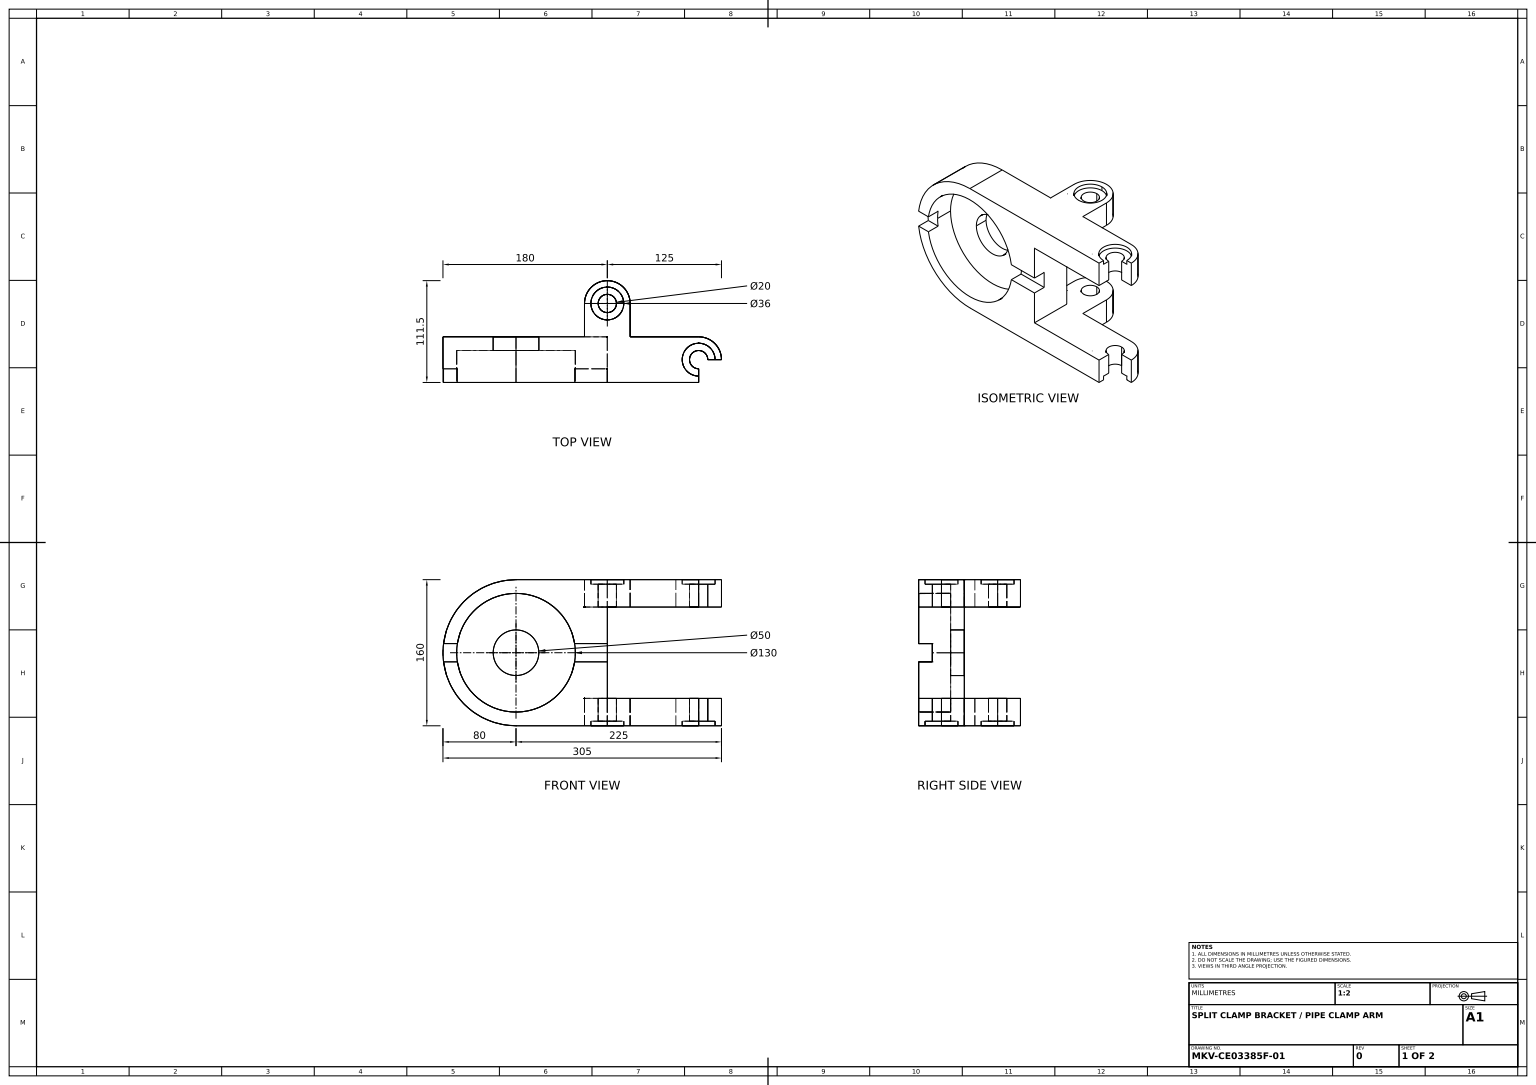
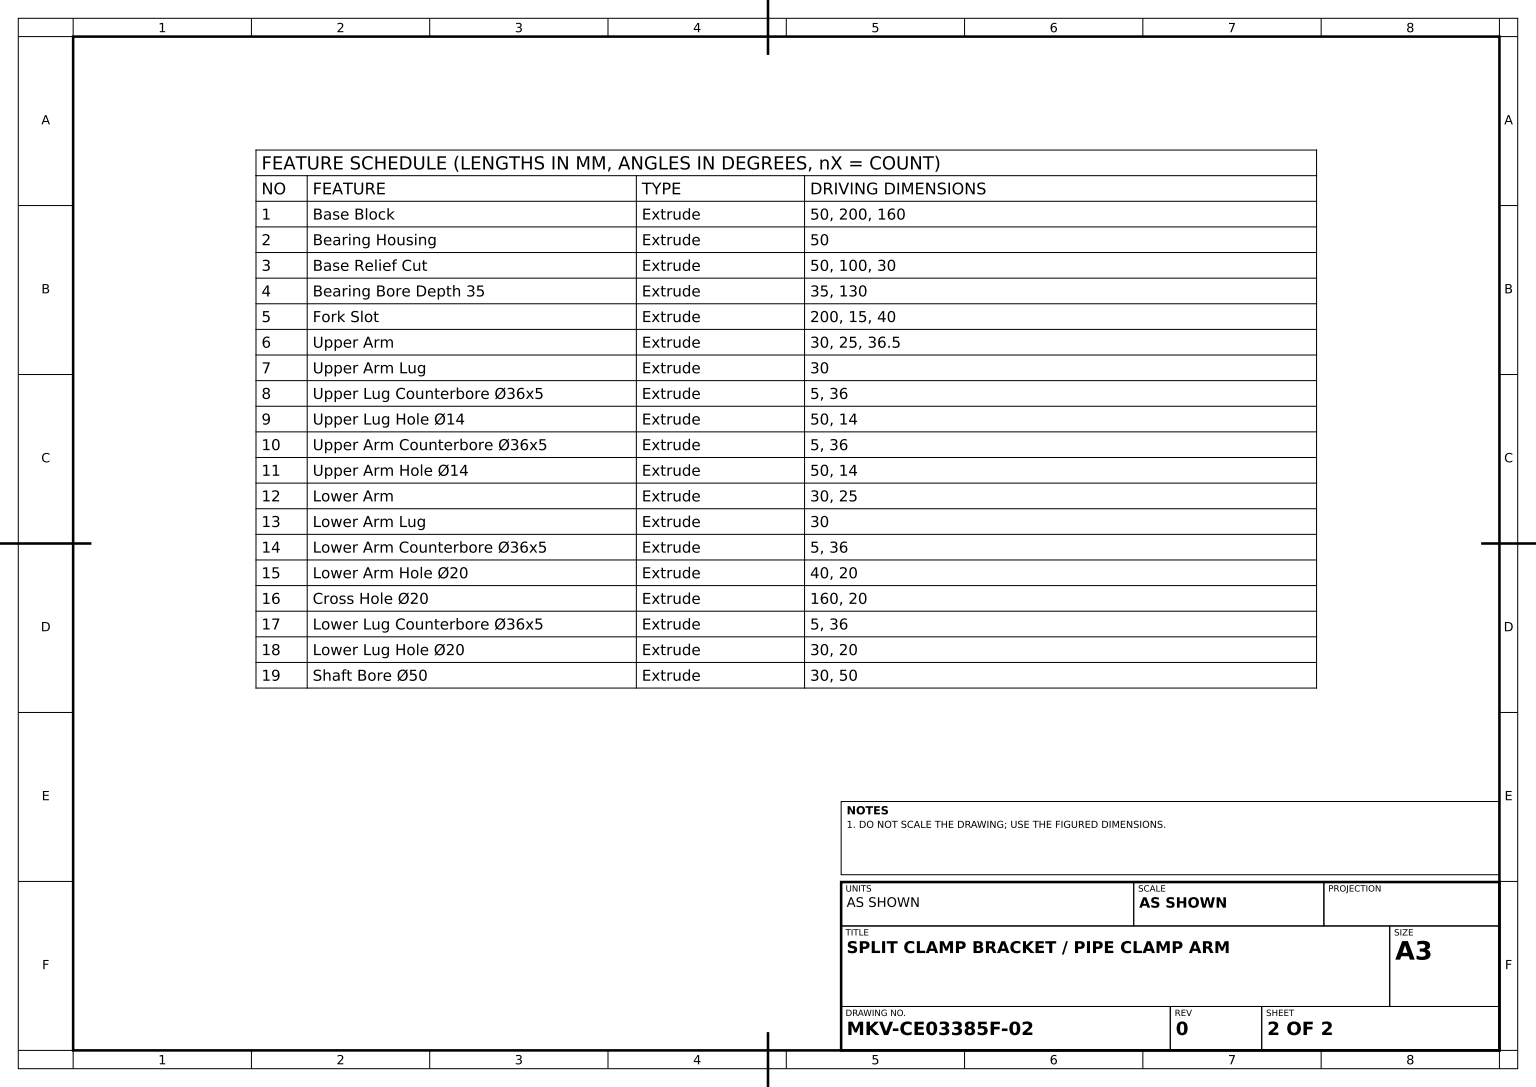
ISO-10303-21;
HEADER;
FILE_DESCRIPTION((''),'2;1');
FILE_NAME('','',(''),(''),'','','');
FILE_SCHEMA(('AUTOMOTIVE_DESIGN'));
ENDSEC;
DATA;
#1=APPLICATION_CONTEXT('');
#2=PRODUCT_CONTEXT('',#1,'mechanical');
#3=PRODUCT('','','',(#2));
#4=PRODUCT_DEFINITION_FORMATION('','',#3);
#5=PRODUCT_DEFINITION_CONTEXT('',#1,'design');
#6=PRODUCT_DEFINITION('','',#4,#5);
#7=PRODUCT_DEFINITION_SHAPE('','',#6);
#8=(LENGTH_UNIT()NAMED_UNIT(*)SI_UNIT(.MILLI.,.METRE.));
#9=(NAMED_UNIT(*)PLANE_ANGLE_UNIT()SI_UNIT($,.RADIAN.));
#10=(NAMED_UNIT(*)SI_UNIT($,.STERADIAN.)SOLID_ANGLE_UNIT());
#11=UNCERTAINTY_MEASURE_WITH_UNIT(LENGTH_MEASURE(1.E-05),#8,'distance_accuracy_value','');
#12=(GEOMETRIC_REPRESENTATION_CONTEXT(3)GLOBAL_UNCERTAINTY_ASSIGNED_CONTEXT((#11))GLOBAL_UNIT_ASSIGNED_CONTEXT((#8,#9,#10))REPRESENTATION_CONTEXT('',''));
#13=CARTESIAN_POINT('',(100.,130.,-26.5));
#14=VERTEX_POINT('',#13);
#15=CARTESIAN_POINT('',(100.,130.,-46.5));
#16=VERTEX_POINT('',#15);
#17=CARTESIAN_POINT('',(100.,130.,-36.5));
#18=DIRECTION('',(0.,1.,0.));
#19=DIRECTION('',(0.,0.,1.));
#20=AXIS2_PLACEMENT_3D('',#17,#18,#19);
#21=CIRCLE('',#20,10.);
#22=EDGE_CURVE('',#14,#16,#21,.T.);
#23=ORIENTED_EDGE('',*,*,#22,.T.);
#24=EDGE_CURVE('',#16,#14,#21,.T.);
#25=ORIENTED_EDGE('',*,*,#24,.T.);
#26=EDGE_LOOP('',(#23,#25));
#27=FACE_BOUND('',#26,.T.);
#28=CARTESIAN_POINT('',(100.,130.,0.));
#29=VERTEX_POINT('',#28);
#30=CARTESIAN_POINT('',(100.,130.,50.));
#31=VERTEX_POINT('',#30);
#32=VECTOR('',#19,1000.);
#33=LINE('',#28,#32);
#34=EDGE_CURVE('',#29,#31,#33,.T.);
#35=ORIENTED_EDGE('',*,*,#34,.F.);
#36=CARTESIAN_POINT('',(75.,130.,0.));
#37=VERTEX_POINT('',#36);
#38=CARTESIAN_POINT('',(125.,130.,0.));
#39=DIRECTION('',(1.,0.,0.));
#40=VECTOR('',#39,1000.);
#41=LINE('',#38,#40);
#42=EDGE_CURVE('',#37,#29,#41,.T.);
#43=ORIENTED_EDGE('',*,*,#42,.F.);
#44=CARTESIAN_POINT('',(75.,130.,-36.5));
#45=VERTEX_POINT('',#44);
#46=LINE('',#44,#32);
#47=EDGE_CURVE('',#45,#37,#46,.T.);
#48=ORIENTED_EDGE('',*,*,#47,.F.);
#49=CARTESIAN_POINT('',(125.,130.,-36.5));
#50=VERTEX_POINT('',#49);
#51=CIRCLE('',#20,25.);
#52=EDGE_CURVE('',#50,#45,#51,.T.);
#53=ORIENTED_EDGE('',*,*,#52,.F.);
#54=VERTEX_POINT('',#38);
#55=DIRECTION('',(0.,0.,-1.));
#56=VECTOR('',#55,1000.);
#57=LINE('',#49,#56);
#58=EDGE_CURVE('',#54,#50,#57,.T.);
#59=ORIENTED_EDGE('',*,*,#58,.F.);
#60=CARTESIAN_POINT('',(200.,130.,0.));
#61=VERTEX_POINT('',#60);
#62=DIRECTION('',(-1.,0.,0.));
#63=VECTOR('',#62,1000.);
#64=LINE('',#60,#63);
#65=EDGE_CURVE('',#61,#54,#64,.T.);
#66=ORIENTED_EDGE('',*,*,#65,.F.);
#67=CARTESIAN_POINT('',(225.,130.,25.));
#68=VERTEX_POINT('',#67);
#69=CARTESIAN_POINT('',(200.,130.,25.));
#70=AXIS2_PLACEMENT_3D('',#69,#18,#19);
#71=CIRCLE('',#70,25.);
#72=EDGE_CURVE('',#68,#61,#71,.T.);
#73=ORIENTED_EDGE('',*,*,#72,.F.);
#74=CARTESIAN_POINT('',(210.,130.,25.));
#75=VERTEX_POINT('',#74);
#76=LINE('',#69,#40);
#77=EDGE_CURVE('',#75,#68,#76,.T.);
#78=ORIENTED_EDGE('',*,*,#77,.F.);
#79=CARTESIAN_POINT('',(200.,130.,35.));
#80=VERTEX_POINT('',#79);
#81=CIRCLE('',#70,10.);
#82=EDGE_CURVE('',#75,#80,#81,.T.);
#83=ORIENTED_EDGE('',*,*,#82,.T.);
#84=CARTESIAN_POINT('',(200.,130.,50.));
#85=VERTEX_POINT('',#84);
#86=LINE('',#60,#32);
#87=EDGE_CURVE('',#80,#85,#86,.T.);
#88=ORIENTED_EDGE('',*,*,#87,.T.);
#89=LINE('',#84,#63);
#90=EDGE_CURVE('',#85,#31,#89,.T.);
#91=ORIENTED_EDGE('',*,*,#90,.T.);
#92=EDGE_LOOP('',(#35,#43,#48,#53,#59,#66,#73,#78,#83,#88,#91));
#93=FACE_OUTER_BOUND('',#92,.T.);
#94=AXIS2_PLACEMENT_3D('',#60,#18,#19);
#95=PLANE('',#94);
#96=ADVANCED_FACE('',(#27,#93),#95,.F.);
#97=ORIENTED_EDGE('',*,*,#52,.T.);
#98=CARTESIAN_POINT('',(75.,160.,-36.5));
#99=VERTEX_POINT('',#98);
#100=VECTOR('',#18,1000.);
#101=LINE('',#44,#100);
#102=EDGE_CURVE('',#45,#99,#101,.T.);
#103=ORIENTED_EDGE('',*,*,#102,.T.);
#104=CARTESIAN_POINT('',(125.,160.,-36.5));
#105=VERTEX_POINT('',#104);
#106=CARTESIAN_POINT('',(100.,160.,-36.5));
#107=AXIS2_PLACEMENT_3D('',#106,#18,#19);
#108=CIRCLE('',#107,25.);
#109=EDGE_CURVE('',#105,#99,#108,.T.);
#110=ORIENTED_EDGE('',*,*,#109,.F.);
#111=LINE('',#49,#100);
#112=EDGE_CURVE('',#50,#105,#111,.T.);
#113=ORIENTED_EDGE('',*,*,#112,.F.);
#114=EDGE_LOOP('',(#97,#103,#110,#113));
#115=FACE_OUTER_BOUND('',#114,.T.);
#116=CYLINDRICAL_SURFACE('',#20,25.);
#117=ADVANCED_FACE('',(#115),#116,.T.);
#118=CARTESIAN_POINT('',(200.,30.,0.));
#119=VERTEX_POINT('',#118);
#120=CARTESIAN_POINT('',(225.,30.,25.));
#121=VERTEX_POINT('',#120);
#122=CARTESIAN_POINT('',(200.,30.,25.));
#123=DIRECTION('',(0.,-1.,0.));
#124=AXIS2_PLACEMENT_3D('',#122,#123,#55);
#125=CIRCLE('',#124,25.);
#126=EDGE_CURVE('',#119,#121,#125,.T.);
#127=ORIENTED_EDGE('',*,*,#126,.T.);
#128=CARTESIAN_POINT('',(225.,0.,25.));
#129=VERTEX_POINT('',#128);
#130=VECTOR('',#123,1000.);
#131=LINE('',#120,#130);
#132=EDGE_CURVE('',#121,#129,#131,.T.);
#133=ORIENTED_EDGE('',*,*,#132,.T.);
#134=CARTESIAN_POINT('',(200.,0.,0.));
#135=VERTEX_POINT('',#134);
#136=CARTESIAN_POINT('',(200.,0.,25.));
#137=AXIS2_PLACEMENT_3D('',#136,#123,#55);
#138=CIRCLE('',#137,25.);
#139=EDGE_CURVE('',#135,#129,#138,.T.);
#140=ORIENTED_EDGE('',*,*,#139,.F.);
#141=LINE('',#134,#100);
#142=EDGE_CURVE('',#135,#119,#141,.T.);
#143=ORIENTED_EDGE('',*,*,#142,.T.);
#144=EDGE_LOOP('',(#127,#133,#140,#143));
#145=FACE_OUTER_BOUND('',#144,.T.);
#146=CYLINDRICAL_SURFACE('',#124,25.);
#147=ADVANCED_FACE('',(#145),#146,.T.);
#148=CARTESIAN_POINT('',(200.,5.,35.));
#149=VERTEX_POINT('',#148);
#150=CARTESIAN_POINT('',(200.,30.,35.));
#151=VERTEX_POINT('',#150);
#152=CARTESIAN_POINT('',(200.,45.,35.));
#153=LINE('',#152,#100);
#154=EDGE_CURVE('',#149,#151,#153,.T.);
#155=ORIENTED_EDGE('',*,*,#154,.T.);
#156=CARTESIAN_POINT('',(200.,30.,50.));
#157=VERTEX_POINT('',#156);
#158=LINE('',#118,#32);
#159=EDGE_CURVE('',#151,#157,#158,.T.);
#160=ORIENTED_EDGE('',*,*,#159,.T.);
#161=CARTESIAN_POINT('',(200.,0.,50.));
#162=VERTEX_POINT('',#161);
#163=LINE('',#161,#100);
#164=EDGE_CURVE('',#162,#157,#163,.T.);
#165=ORIENTED_EDGE('',*,*,#164,.F.);
#166=CARTESIAN_POINT('',(200.,0.,43.));
#167=VERTEX_POINT('',#166);
#168=LINE('',#161,#56);
#169=EDGE_CURVE('',#162,#167,#168,.T.);
#170=ORIENTED_EDGE('',*,*,#169,.T.);
#171=CARTESIAN_POINT('',(200.,5.,43.));
#172=VERTEX_POINT('',#171);
#173=LINE('',#171,#100);
#174=EDGE_CURVE('',#167,#172,#173,.T.);
#175=ORIENTED_EDGE('',*,*,#174,.T.);
#176=CARTESIAN_POINT('',(200.,5.,50.));
#177=LINE('',#176,#32);
#178=EDGE_CURVE('',#149,#172,#177,.T.);
#179=ORIENTED_EDGE('',*,*,#178,.F.);
#180=EDGE_LOOP('',(#155,#160,#165,#170,#175,#179));
#181=FACE_OUTER_BOUND('',#180,.T.);
#182=AXIS2_PLACEMENT_3D('',#161,#62,#19);
#183=PLANE('',#182);
#184=ADVANCED_FACE('',(#181),#183,.F.);
#185=CARTESIAN_POINT('',(-79.372539,70.,50.));
#186=VERTEX_POINT('',#185);
#187=CARTESIAN_POINT('',(0.,0.,50.));
#188=VERTEX_POINT('',#187);
#189=CARTESIAN_POINT('',(0.,80.,50.));
#190=AXIS2_PLACEMENT_3D('',#189,#19,#39);
#191=CIRCLE('',#190,80.);
#192=EDGE_CURVE('',#186,#188,#191,.T.);
#193=ORIENTED_EDGE('',*,*,#192,.F.);
#194=CARTESIAN_POINT('',(-79.372539,70.,35.));
#195=VERTEX_POINT('',#194);
#196=CARTESIAN_POINT('',(-79.372539,70.,0.));
#197=LINE('',#196,#32);
#198=EDGE_CURVE('',#195,#186,#197,.T.);
#199=ORIENTED_EDGE('',*,*,#198,.F.);
#200=CARTESIAN_POINT('',(-79.372539,90.,35.));
#201=VERTEX_POINT('',#200);
#202=CARTESIAN_POINT('',(0.,80.,35.));
#203=AXIS2_PLACEMENT_3D('',#202,#19,#62);
#204=CIRCLE('',#203,80.);
#205=EDGE_CURVE('',#201,#195,#204,.T.);
#206=ORIENTED_EDGE('',*,*,#205,.F.);
#207=CARTESIAN_POINT('',(-79.372539,90.,50.));
#208=VERTEX_POINT('',#207);
#209=CARTESIAN_POINT('',(-79.372539,90.,0.));
#210=LINE('',#209,#56);
#211=EDGE_CURVE('',#208,#201,#210,.T.);
#212=ORIENTED_EDGE('',*,*,#211,.F.);
#213=CARTESIAN_POINT('',(0.,160.,50.));
#214=VERTEX_POINT('',#213);
#215=EDGE_CURVE('',#214,#208,#191,.T.);
#216=ORIENTED_EDGE('',*,*,#215,.F.);
#217=CARTESIAN_POINT('',(0.,160.,0.));
#218=VERTEX_POINT('',#217);
#219=LINE('',#213,#56);
#220=EDGE_CURVE('',#214,#218,#219,.T.);
#221=ORIENTED_EDGE('',*,*,#220,.T.);
#222=CARTESIAN_POINT('',(0.,0.,0.));
#223=VERTEX_POINT('',#222);
#224=CARTESIAN_POINT('',(0.,80.,0.));
#225=AXIS2_PLACEMENT_3D('',#224,#19,#39);
#226=CIRCLE('',#225,80.);
#227=EDGE_CURVE('',#218,#223,#226,.T.);
#228=ORIENTED_EDGE('',*,*,#227,.T.);
#229=LINE('',#187,#56);
#230=EDGE_CURVE('',#188,#223,#229,.T.);
#231=ORIENTED_EDGE('',*,*,#230,.F.);
#232=EDGE_LOOP('',(#193,#199,#206,#212,#216,#221,#228,#231));
#233=FACE_OUTER_BOUND('',#232,.T.);
#234=CYLINDRICAL_SURFACE('',#225,80.);
#235=ADVANCED_FACE('',(#233),#234,.T.);
#236=CARTESIAN_POINT('',(75.,0.,0.));
#237=VERTEX_POINT('',#236);
#238=CARTESIAN_POINT('',(75.,0.,-36.5));
#239=VERTEX_POINT('',#238);
#240=LINE('',#238,#56);
#241=EDGE_CURVE('',#237,#239,#240,.T.);
#242=ORIENTED_EDGE('',*,*,#241,.F.);
#243=CARTESIAN_POINT('',(75.,30.,0.));
#244=VERTEX_POINT('',#243);
#245=LINE('',#243,#130);
#246=EDGE_CURVE('',#244,#237,#245,.T.);
#247=ORIENTED_EDGE('',*,*,#246,.F.);
#248=CARTESIAN_POINT('',(75.,30.,-36.5));
#249=VERTEX_POINT('',#248);
#250=LINE('',#248,#56);
#251=EDGE_CURVE('',#244,#249,#250,.T.);
#252=ORIENTED_EDGE('',*,*,#251,.T.);
#253=LINE('',#248,#130);
#254=EDGE_CURVE('',#249,#239,#253,.T.);
#255=ORIENTED_EDGE('',*,*,#254,.T.);
#256=EDGE_LOOP('',(#242,#247,#252,#255));
#257=FACE_OUTER_BOUND('',#256,.T.);
#258=AXIS2_PLACEMENT_3D('',#248,#62,#19);
#259=PLANE('',#258);
#260=ADVANCED_FACE('',(#257),#259,.T.);
#261=CARTESIAN_POINT('',(125.,160.,0.));
#262=VERTEX_POINT('',#261);
#263=LINE('',#38,#100);
#264=EDGE_CURVE('',#54,#262,#263,.T.);
#265=ORIENTED_EDGE('',*,*,#264,.T.);
#266=CARTESIAN_POINT('',(200.,160.,0.));
#267=VERTEX_POINT('',#266);
#268=LINE('',#266,#63);
#269=EDGE_CURVE('',#267,#262,#268,.T.);
#270=ORIENTED_EDGE('',*,*,#269,.F.);
#271=EDGE_CURVE('',#61,#267,#141,.T.);
#272=ORIENTED_EDGE('',*,*,#271,.F.);
#273=ORIENTED_EDGE('',*,*,#65,.T.);
#274=EDGE_LOOP('',(#265,#270,#272,#273));
#275=FACE_OUTER_BOUND('',#274,.T.);
#276=AXIS2_PLACEMENT_3D('',#222,#19,#39);
#277=PLANE('',#276);
#278=ADVANCED_FACE('',(#275),#277,.F.);
#279=CARTESIAN_POINT('',(200.,5.,7.));
#280=VERTEX_POINT('',#279);
#281=CARTESIAN_POINT('',(200.,0.,7.));
#282=VERTEX_POINT('',#281);
#283=LINE('',#279,#130);
#284=EDGE_CURVE('',#280,#282,#283,.T.);
#285=ORIENTED_EDGE('',*,*,#284,.F.);
#286=CARTESIAN_POINT('',(200.,5.,25.));
#287=AXIS2_PLACEMENT_3D('',#286,#123,#55);
#288=CIRCLE('',#287,18.);
#289=EDGE_CURVE('',#172,#280,#288,.T.);
#290=ORIENTED_EDGE('',*,*,#289,.F.);
#291=ORIENTED_EDGE('',*,*,#174,.F.);
#292=CIRCLE('',#137,18.);
#293=EDGE_CURVE('',#167,#282,#292,.T.);
#294=ORIENTED_EDGE('',*,*,#293,.T.);
#295=EDGE_LOOP('',(#285,#290,#291,#294));
#296=FACE_OUTER_BOUND('',#295,.T.);
#297=CYLINDRICAL_SURFACE('',#287,18.);
#298=ADVANCED_FACE('',(#296),#297,.F.);
#299=ORIENTED_EDGE('',*,*,#289,.T.);
#300=CARTESIAN_POINT('',(218.,5.,25.));
#301=VERTEX_POINT('',#300);
#302=EDGE_CURVE('',#280,#301,#288,.T.);
#303=ORIENTED_EDGE('',*,*,#302,.T.);
#304=CARTESIAN_POINT('',(210.,5.,25.));
#305=VERTEX_POINT('',#304);
#306=CARTESIAN_POINT('',(225.,5.,25.));
#307=LINE('',#306,#40);
#308=EDGE_CURVE('',#305,#301,#307,.T.);
#309=ORIENTED_EDGE('',*,*,#308,.F.);
#310=CARTESIAN_POINT('',(200.,5.,15.));
#311=VERTEX_POINT('',#310);
#312=CIRCLE('',#287,10.);
#313=EDGE_CURVE('',#311,#305,#312,.T.);
#314=ORIENTED_EDGE('',*,*,#313,.F.);
#315=EDGE_CURVE('',#149,#311,#312,.T.);
#316=ORIENTED_EDGE('',*,*,#315,.F.);
#317=ORIENTED_EDGE('',*,*,#178,.T.);
#318=EDGE_LOOP('',(#299,#303,#309,#314,#316,#317));
#319=FACE_OUTER_BOUND('',#318,.T.);
#320=PLANE('',#287);
#321=ADVANCED_FACE('',(#319),#320,.T.);
#322=CARTESIAN_POINT('',(-25.,80.,0.));
#323=VERTEX_POINT('',#322);
#324=CARTESIAN_POINT('',(25.,80.,0.));
#325=VERTEX_POINT('',#324);
#326=CIRCLE('',#225,25.);
#327=EDGE_CURVE('',#323,#325,#326,.T.);
#328=ORIENTED_EDGE('',*,*,#327,.T.);
#329=EDGE_CURVE('',#325,#323,#326,.T.);
#330=ORIENTED_EDGE('',*,*,#329,.T.);
#331=EDGE_LOOP('',(#328,#330));
#332=FACE_BOUND('',#331,.T.);
#333=LINE('',#222,#40);
#334=EDGE_CURVE('',#223,#237,#333,.T.);
#335=ORIENTED_EDGE('',*,*,#334,.F.);
#336=ORIENTED_EDGE('',*,*,#227,.F.);
#337=CARTESIAN_POINT('',(75.,160.,0.));
#338=VERTEX_POINT('',#337);
#339=EDGE_CURVE('',#338,#218,#268,.T.);
#340=ORIENTED_EDGE('',*,*,#339,.F.);
#341=LINE('',#36,#100);
#342=EDGE_CURVE('',#37,#338,#341,.T.);
#343=ORIENTED_EDGE('',*,*,#342,.F.);
#344=ORIENTED_EDGE('',*,*,#42,.T.);
#345=CARTESIAN_POINT('',(100.,30.,0.));
#346=VERTEX_POINT('',#345);
#347=LINE('',#28,#130);
#348=EDGE_CURVE('',#29,#346,#347,.T.);
#349=ORIENTED_EDGE('',*,*,#348,.T.);
#350=LINE('',#243,#63);
#351=EDGE_CURVE('',#346,#244,#350,.T.);
#352=ORIENTED_EDGE('',*,*,#351,.T.);
#353=ORIENTED_EDGE('',*,*,#246,.T.);
#354=EDGE_LOOP('',(#335,#336,#340,#343,#344,#349,#352,#353));
#355=FACE_OUTER_BOUND('',#354,.T.);
#356=ADVANCED_FACE('',(#332,#355),#277,.F.);
#357=CARTESIAN_POINT('',(-64.226163,90.,50.));
#358=VERTEX_POINT('',#357);
#359=CARTESIAN_POINT('',(-100.,90.,50.));
#360=LINE('',#359,#40);
#361=EDGE_CURVE('',#208,#358,#360,.T.);
#362=ORIENTED_EDGE('',*,*,#361,.F.);
#363=ORIENTED_EDGE('',*,*,#211,.T.);
#364=CARTESIAN_POINT('',(-64.226163,90.,35.));
#365=VERTEX_POINT('',#364);
#366=CARTESIAN_POINT('',(-100.,90.,35.));
#367=LINE('',#366,#40);
#368=EDGE_CURVE('',#201,#365,#367,.T.);
#369=ORIENTED_EDGE('',*,*,#368,.T.);
#370=CARTESIAN_POINT('',(-64.226163,90.,15.));
#371=LINE('',#370,#56);
#372=EDGE_CURVE('',#358,#365,#371,.T.);
#373=ORIENTED_EDGE('',*,*,#372,.F.);
#374=EDGE_LOOP('',(#362,#363,#369,#373));
#375=FACE_OUTER_BOUND('',#374,.T.);
#376=AXIS2_PLACEMENT_3D('',#359,#18,#19);
#377=PLANE('',#376);
#378=ADVANCED_FACE('',(#375),#377,.F.);
#379=CARTESIAN_POINT('',(100.,155.,-18.5));
#380=VERTEX_POINT('',#379);
#381=CARTESIAN_POINT('',(100.,160.,-18.5));
#382=VERTEX_POINT('',#381);
#383=LINE('',#379,#100);
#384=EDGE_CURVE('',#380,#382,#383,.T.);
#385=ORIENTED_EDGE('',*,*,#384,.F.);
#386=CARTESIAN_POINT('',(100.,155.,-54.5));
#387=VERTEX_POINT('',#386);
#388=CARTESIAN_POINT('',(100.,155.,-36.5));
#389=AXIS2_PLACEMENT_3D('',#388,#18,#19);
#390=CIRCLE('',#389,18.);
#391=EDGE_CURVE('',#387,#380,#390,.T.);
#392=ORIENTED_EDGE('',*,*,#391,.F.);
#393=CARTESIAN_POINT('',(100.,160.,-54.5));
#394=VERTEX_POINT('',#393);
#395=LINE('',#386,#100);
#396=EDGE_CURVE('',#387,#394,#395,.T.);
#397=ORIENTED_EDGE('',*,*,#396,.T.);
#398=CIRCLE('',#107,18.);
#399=EDGE_CURVE('',#394,#382,#398,.T.);
#400=ORIENTED_EDGE('',*,*,#399,.T.);
#401=EDGE_LOOP('',(#385,#392,#397,#400));
#402=FACE_OUTER_BOUND('',#401,.T.);
#403=CYLINDRICAL_SURFACE('',#389,18.);
#404=ADVANCED_FACE('',(#402),#403,.F.);
#405=ORIENTED_EDGE('',*,*,#302,.F.);
#406=ORIENTED_EDGE('',*,*,#284,.T.);
#407=CARTESIAN_POINT('',(218.,0.,25.));
#408=VERTEX_POINT('',#407);
#409=EDGE_CURVE('',#282,#408,#292,.T.);
#410=ORIENTED_EDGE('',*,*,#409,.T.);
#411=LINE('',#300,#100);
#412=EDGE_CURVE('',#408,#301,#411,.T.);
#413=ORIENTED_EDGE('',*,*,#412,.T.);
#414=EDGE_LOOP('',(#405,#406,#410,#413));
#415=FACE_OUTER_BOUND('',#414,.T.);
#416=ADVANCED_FACE('',(#415),#297,.F.);
#417=ORIENTED_EDGE('',*,*,#198,.T.);
#418=CARTESIAN_POINT('',(-64.226163,70.,50.));
#419=VERTEX_POINT('',#418);
#420=CARTESIAN_POINT('',(-100.,70.,50.));
#421=LINE('',#420,#40);
#422=EDGE_CURVE('',#186,#419,#421,.T.);
#423=ORIENTED_EDGE('',*,*,#422,.T.);
#424=CARTESIAN_POINT('',(-64.226163,70.,35.));
#425=VERTEX_POINT('',#424);
#426=CARTESIAN_POINT('',(-64.226163,70.,15.));
#427=LINE('',#426,#32);
#428=EDGE_CURVE('',#425,#419,#427,.T.);
#429=ORIENTED_EDGE('',*,*,#428,.F.);
#430=CARTESIAN_POINT('',(-100.,70.,35.));
#431=LINE('',#430,#40);
#432=EDGE_CURVE('',#195,#425,#431,.T.);
#433=ORIENTED_EDGE('',*,*,#432,.F.);
#434=EDGE_LOOP('',(#417,#423,#429,#433));
#435=FACE_OUTER_BOUND('',#434,.T.);
#436=AXIS2_PLACEMENT_3D('',#430,#123,#55);
#437=PLANE('',#436);
#438=ADVANCED_FACE('',(#435),#437,.F.);
#439=CARTESIAN_POINT('',(100.,155.,-26.5));
#440=VERTEX_POINT('',#439);
#441=CARTESIAN_POINT('',(100.,165.,-26.5));
#442=LINE('',#441,#130);
#443=EDGE_CURVE('',#440,#14,#442,.T.);
#444=ORIENTED_EDGE('',*,*,#443,.T.);
#445=ORIENTED_EDGE('',*,*,#24,.F.);
#446=CARTESIAN_POINT('',(100.,155.,-46.5));
#447=VERTEX_POINT('',#446);
#448=CARTESIAN_POINT('',(100.,165.,-46.5));
#449=LINE('',#448,#130);
#450=EDGE_CURVE('',#447,#16,#449,.T.);
#451=ORIENTED_EDGE('',*,*,#450,.F.);
#452=CIRCLE('',#389,10.);
#453=EDGE_CURVE('',#447,#440,#452,.T.);
#454=ORIENTED_EDGE('',*,*,#453,.T.);
#455=EDGE_LOOP('',(#444,#445,#451,#454));
#456=FACE_OUTER_BOUND('',#455,.T.);
#457=CARTESIAN_POINT('',(100.,165.,-36.5));
#458=AXIS2_PLACEMENT_3D('',#457,#123,#55);
#459=CYLINDRICAL_SURFACE('',#458,10.);
#460=ADVANCED_FACE('',(#456),#459,.F.);
#461=CARTESIAN_POINT('',(64.226163,70.,50.));
#462=VERTEX_POINT('',#461);
#463=CIRCLE('',#190,65.);
#464=EDGE_CURVE('',#419,#462,#463,.T.);
#465=ORIENTED_EDGE('',*,*,#464,.T.);
#466=CARTESIAN_POINT('',(64.226163,70.,35.));
#467=VERTEX_POINT('',#466);
#468=CARTESIAN_POINT('',(64.226163,70.,15.));
#469=LINE('',#468,#56);
#470=EDGE_CURVE('',#462,#467,#469,.T.);
#471=ORIENTED_EDGE('',*,*,#470,.T.);
#472=CARTESIAN_POINT('',(65.,80.,35.));
#473=VERTEX_POINT('',#472);
#474=CIRCLE('',#203,65.);
#475=EDGE_CURVE('',#467,#473,#474,.T.);
#476=ORIENTED_EDGE('',*,*,#475,.T.);
#477=CARTESIAN_POINT('',(65.,80.,15.));
#478=VERTEX_POINT('',#477);
#479=LINE('',#477,#32);
#480=EDGE_CURVE('',#478,#473,#479,.T.);
#481=ORIENTED_EDGE('',*,*,#480,.F.);
#482=CARTESIAN_POINT('',(-65.,80.,15.));
#483=VERTEX_POINT('',#482);
#484=CARTESIAN_POINT('',(0.,80.,15.));
#485=AXIS2_PLACEMENT_3D('',#484,#19,#39);
#486=CIRCLE('',#485,65.);
#487=EDGE_CURVE('',#483,#478,#486,.T.);
#488=ORIENTED_EDGE('',*,*,#487,.F.);
#489=CARTESIAN_POINT('',(-65.,80.,35.));
#490=VERTEX_POINT('',#489);
#491=LINE('',#482,#32);
#492=EDGE_CURVE('',#483,#490,#491,.T.);
#493=ORIENTED_EDGE('',*,*,#492,.T.);
#494=EDGE_CURVE('',#490,#425,#474,.T.);
#495=ORIENTED_EDGE('',*,*,#494,.T.);
#496=ORIENTED_EDGE('',*,*,#428,.T.);
#497=EDGE_LOOP('',(#465,#471,#476,#481,#488,#493,#495,#496));
#498=FACE_OUTER_BOUND('',#497,.T.);
#499=CYLINDRICAL_SURFACE('',#485,65.);
#500=ADVANCED_FACE('',(#498),#499,.F.);
#501=CARTESIAN_POINT('',(200.,155.,43.));
#502=VERTEX_POINT('',#501);
#503=CARTESIAN_POINT('',(200.,160.,43.));
#504=VERTEX_POINT('',#503);
#505=LINE('',#501,#100);
#506=EDGE_CURVE('',#502,#504,#505,.T.);
#507=ORIENTED_EDGE('',*,*,#506,.T.);
#508=CARTESIAN_POINT('',(200.,160.,50.));
#509=VERTEX_POINT('',#508);
#510=LINE('',#508,#56);
#511=EDGE_CURVE('',#509,#504,#510,.T.);
#512=ORIENTED_EDGE('',*,*,#511,.F.);
#513=EDGE_CURVE('',#85,#509,#163,.T.);
#514=ORIENTED_EDGE('',*,*,#513,.F.);
#515=ORIENTED_EDGE('',*,*,#87,.F.);
#516=CARTESIAN_POINT('',(200.,155.,35.));
#517=VERTEX_POINT('',#516);
#518=LINE('',#79,#100);
#519=EDGE_CURVE('',#80,#517,#518,.T.);
#520=ORIENTED_EDGE('',*,*,#519,.T.);
#521=CARTESIAN_POINT('',(200.,155.,50.));
#522=LINE('',#521,#56);
#523=EDGE_CURVE('',#502,#517,#522,.T.);
#524=ORIENTED_EDGE('',*,*,#523,.F.);
#525=EDGE_LOOP('',(#507,#512,#514,#515,#520,#524));
#526=FACE_OUTER_BOUND('',#525,.T.);
#527=ADVANCED_FACE('',(#526),#183,.F.);
#528=CARTESIAN_POINT('',(100.,70.,50.));
#529=VERTEX_POINT('',#528);
#530=CARTESIAN_POINT('',(100.,30.,50.));
#531=VERTEX_POINT('',#530);
#532=LINE('',#30,#130);
#533=EDGE_CURVE('',#529,#531,#532,.T.);
#534=ORIENTED_EDGE('',*,*,#533,.T.);
#535=LINE('',#345,#32);
#536=EDGE_CURVE('',#346,#531,#535,.T.);
#537=ORIENTED_EDGE('',*,*,#536,.F.);
#538=ORIENTED_EDGE('',*,*,#348,.F.);
#539=ORIENTED_EDGE('',*,*,#34,.T.);
#540=CARTESIAN_POINT('',(100.,90.,50.));
#541=VERTEX_POINT('',#540);
#542=EDGE_CURVE('',#31,#541,#532,.T.);
#543=ORIENTED_EDGE('',*,*,#542,.T.);
#544=CARTESIAN_POINT('',(100.,90.,35.));
#545=VERTEX_POINT('',#544);
#546=LINE('',#540,#32);
#547=EDGE_CURVE('',#545,#541,#546,.T.);
#548=ORIENTED_EDGE('',*,*,#547,.F.);
#549=CARTESIAN_POINT('',(100.,70.,35.));
#550=VERTEX_POINT('',#549);
#551=LINE('',#544,#100);
#552=EDGE_CURVE('',#550,#545,#551,.T.);
#553=ORIENTED_EDGE('',*,*,#552,.F.);
#554=LINE('',#549,#56);
#555=EDGE_CURVE('',#529,#550,#554,.T.);
#556=ORIENTED_EDGE('',*,*,#555,.F.);
#557=EDGE_LOOP('',(#534,#537,#538,#539,#543,#548,#553,#556));
#558=FACE_OUTER_BOUND('',#557,.T.);
#559=AXIS2_PLACEMENT_3D('',#28,#62,#19);
#560=PLANE('',#559);
#561=ADVANCED_FACE('',(#558),#560,.F.);
#562=ORIENTED_EDGE('',*,*,#264,.F.);
#563=ORIENTED_EDGE('',*,*,#58,.T.);
#564=ORIENTED_EDGE('',*,*,#112,.T.);
#565=LINE('',#104,#56);
#566=EDGE_CURVE('',#262,#105,#565,.T.);
#567=ORIENTED_EDGE('',*,*,#566,.F.);
#568=EDGE_LOOP('',(#562,#563,#564,#567));
#569=FACE_OUTER_BOUND('',#568,.T.);
#570=AXIS2_PLACEMENT_3D('',#49,#39,#55);
#571=PLANE('',#570);
#572=ADVANCED_FACE('',(#569),#571,.T.);
#573=CARTESIAN_POINT('',(100.,5.,-54.5));
#574=VERTEX_POINT('',#573);
#575=CARTESIAN_POINT('',(100.,5.,-18.5));
#576=VERTEX_POINT('',#575);
#577=CARTESIAN_POINT('',(100.,5.,-36.5));
#578=AXIS2_PLACEMENT_3D('',#577,#123,#55);
#579=CIRCLE('',#578,18.);
#580=EDGE_CURVE('',#574,#576,#579,.T.);
#581=ORIENTED_EDGE('',*,*,#580,.F.);
#582=CARTESIAN_POINT('',(100.,0.,-54.5));
#583=VERTEX_POINT('',#582);
#584=LINE('',#573,#130);
#585=EDGE_CURVE('',#574,#583,#584,.T.);
#586=ORIENTED_EDGE('',*,*,#585,.T.);
#587=CARTESIAN_POINT('',(100.,0.,-18.5));
#588=VERTEX_POINT('',#587);
#589=CARTESIAN_POINT('',(100.,0.,-36.5));
#590=AXIS2_PLACEMENT_3D('',#589,#123,#55);
#591=CIRCLE('',#590,18.);
#592=EDGE_CURVE('',#583,#588,#591,.T.);
#593=ORIENTED_EDGE('',*,*,#592,.T.);
#594=LINE('',#575,#130);
#595=EDGE_CURVE('',#576,#588,#594,.T.);
#596=ORIENTED_EDGE('',*,*,#595,.F.);
#597=EDGE_LOOP('',(#581,#586,#593,#596));
#598=FACE_OUTER_BOUND('',#597,.T.);
#599=CYLINDRICAL_SURFACE('',#578,18.);
#600=ADVANCED_FACE('',(#598),#599,.F.);
#601=ORIENTED_EDGE('',*,*,#313,.T.);
#602=CARTESIAN_POINT('',(210.,30.,25.));
#603=VERTEX_POINT('',#602);
#604=CARTESIAN_POINT('',(210.,45.,25.));
#605=LINE('',#604,#100);
#606=EDGE_CURVE('',#305,#603,#605,.T.);
#607=ORIENTED_EDGE('',*,*,#606,.T.);
#608=CARTESIAN_POINT('',(200.,30.,15.));
#609=VERTEX_POINT('',#608);
#610=CIRCLE('',#124,10.);
#611=EDGE_CURVE('',#609,#603,#610,.T.);
#612=ORIENTED_EDGE('',*,*,#611,.F.);
#613=CARTESIAN_POINT('',(200.,45.,15.));
#614=LINE('',#613,#130);
#615=EDGE_CURVE('',#609,#311,#614,.T.);
#616=ORIENTED_EDGE('',*,*,#615,.T.);
#617=EDGE_LOOP('',(#601,#607,#612,#616));
#618=FACE_OUTER_BOUND('',#617,.T.);
#619=CARTESIAN_POINT('',(200.,45.,25.));
#620=AXIS2_PLACEMENT_3D('',#619,#123,#55);
#621=CYLINDRICAL_SURFACE('',#620,10.);
#622=ADVANCED_FACE('',(#618),#621,.F.);
#623=CARTESIAN_POINT('',(210.,155.,25.));
#624=VERTEX_POINT('',#623);
#625=CARTESIAN_POINT('',(200.,155.,25.));
#626=AXIS2_PLACEMENT_3D('',#625,#18,#19);
#627=CIRCLE('',#626,10.);
#628=EDGE_CURVE('',#624,#517,#627,.T.);
#629=ORIENTED_EDGE('',*,*,#628,.T.);
#630=ORIENTED_EDGE('',*,*,#519,.F.);
#631=ORIENTED_EDGE('',*,*,#82,.F.);
#632=LINE('',#74,#100);
#633=EDGE_CURVE('',#75,#624,#632,.T.);
#634=ORIENTED_EDGE('',*,*,#633,.T.);
#635=EDGE_LOOP('',(#629,#630,#631,#634));
#636=FACE_OUTER_BOUND('',#635,.T.);
#637=CYLINDRICAL_SURFACE('',#70,10.);
#638=ADVANCED_FACE('',(#636),#637,.F.);
#639=CARTESIAN_POINT('',(125.,30.,0.));
#640=VERTEX_POINT('',#639);
#641=CARTESIAN_POINT('',(125.,0.,0.));
#642=VERTEX_POINT('',#641);
#643=LINE('',#639,#130);
#644=EDGE_CURVE('',#640,#642,#643,.T.);
#645=ORIENTED_EDGE('',*,*,#644,.F.);
#646=LINE('',#345,#40);
#647=EDGE_CURVE('',#640,#119,#646,.T.);
#648=ORIENTED_EDGE('',*,*,#647,.T.);
#649=ORIENTED_EDGE('',*,*,#142,.F.);
#650=EDGE_CURVE('',#642,#135,#333,.T.);
#651=ORIENTED_EDGE('',*,*,#650,.F.);
#652=EDGE_LOOP('',(#645,#648,#649,#651));
#653=FACE_OUTER_BOUND('',#652,.T.);
#654=ADVANCED_FACE('',(#653),#277,.F.);
#655=CARTESIAN_POINT('',(225.,160.,25.));
#656=VERTEX_POINT('',#655);
#657=LINE('',#67,#100);
#658=EDGE_CURVE('',#68,#656,#657,.T.);
#659=ORIENTED_EDGE('',*,*,#658,.F.);
#660=ORIENTED_EDGE('',*,*,#72,.T.);
#661=ORIENTED_EDGE('',*,*,#271,.T.);
#662=CARTESIAN_POINT('',(200.,160.,25.));
#663=AXIS2_PLACEMENT_3D('',#662,#18,#19);
#664=CIRCLE('',#663,25.);
#665=EDGE_CURVE('',#656,#267,#664,.T.);
#666=ORIENTED_EDGE('',*,*,#665,.F.);
#667=EDGE_LOOP('',(#659,#660,#661,#666));
#668=FACE_OUTER_BOUND('',#667,.T.);
#669=CYLINDRICAL_SURFACE('',#70,25.);
#670=ADVANCED_FACE('',(#668),#669,.T.);
#671=EDGE_CURVE('',#382,#394,#398,.T.);
#672=ORIENTED_EDGE('',*,*,#671,.F.);
#673=ORIENTED_EDGE('',*,*,#399,.F.);
#674=EDGE_LOOP('',(#672,#673));
#675=FACE_BOUND('',#674,.T.);
#676=ORIENTED_EDGE('',*,*,#339,.T.);
#677=ORIENTED_EDGE('',*,*,#220,.F.);
#678=LINE('',#508,#63);
#679=EDGE_CURVE('',#509,#214,#678,.T.);
#680=ORIENTED_EDGE('',*,*,#679,.F.);
#681=ORIENTED_EDGE('',*,*,#511,.T.);
#682=CARTESIAN_POINT('',(218.,160.,25.));
#683=VERTEX_POINT('',#682);
#684=CIRCLE('',#663,18.);
#685=EDGE_CURVE('',#683,#504,#684,.T.);
#686=ORIENTED_EDGE('',*,*,#685,.F.);
#687=LINE('',#662,#40);
#688=EDGE_CURVE('',#683,#656,#687,.T.);
#689=ORIENTED_EDGE('',*,*,#688,.T.);
#690=ORIENTED_EDGE('',*,*,#665,.T.);
#691=ORIENTED_EDGE('',*,*,#269,.T.);
#692=ORIENTED_EDGE('',*,*,#566,.T.);
#693=ORIENTED_EDGE('',*,*,#109,.T.);
#694=LINE('',#98,#32);
#695=EDGE_CURVE('',#99,#338,#694,.T.);
#696=ORIENTED_EDGE('',*,*,#695,.T.);
#697=EDGE_LOOP('',(#676,#677,#680,#681,#686,#689,#690,#691,#692,#693,#696));
#698=FACE_OUTER_BOUND('',#697,.T.);
#699=AXIS2_PLACEMENT_3D('',#508,#123,#55);
#700=PLANE('',#699);
#701=ADVANCED_FACE('',(#675,#698),#700,.F.);
#702=ORIENTED_EDGE('',*,*,#126,.F.);
#703=ORIENTED_EDGE('',*,*,#647,.F.);
#704=CARTESIAN_POINT('',(125.,30.,-36.5));
#705=VERTEX_POINT('',#704);
#706=LINE('',#704,#32);
#707=EDGE_CURVE('',#705,#640,#706,.T.);
#708=ORIENTED_EDGE('',*,*,#707,.F.);
#709=CARTESIAN_POINT('',(100.,30.,-61.5));
#710=VERTEX_POINT('',#709);
#711=CARTESIAN_POINT('',(100.,30.,-36.5));
#712=AXIS2_PLACEMENT_3D('',#711,#123,#55);
#713=CIRCLE('',#712,25.);
#714=EDGE_CURVE('',#710,#705,#713,.T.);
#715=ORIENTED_EDGE('',*,*,#714,.F.);
#716=EDGE_CURVE('',#249,#710,#713,.T.);
#717=ORIENTED_EDGE('',*,*,#716,.F.);
#718=ORIENTED_EDGE('',*,*,#251,.F.);
#719=ORIENTED_EDGE('',*,*,#351,.F.);
#720=ORIENTED_EDGE('',*,*,#536,.T.);
#721=LINE('',#530,#40);
#722=EDGE_CURVE('',#531,#157,#721,.T.);
#723=ORIENTED_EDGE('',*,*,#722,.T.);
#724=ORIENTED_EDGE('',*,*,#159,.F.);
#725=EDGE_CURVE('',#151,#609,#610,.T.);
#726=ORIENTED_EDGE('',*,*,#725,.T.);
#727=ORIENTED_EDGE('',*,*,#611,.T.);
#728=LINE('',#120,#63);
#729=EDGE_CURVE('',#121,#603,#728,.T.);
#730=ORIENTED_EDGE('',*,*,#729,.F.);
#731=EDGE_LOOP('',(#702,#703,#708,#715,#717,#718,#719,#720,#723,#724,#726,#727,#730));
#732=FACE_OUTER_BOUND('',#731,.T.);
#733=CARTESIAN_POINT('',(100.,30.,-26.5));
#734=VERTEX_POINT('',#733);
#735=CARTESIAN_POINT('',(100.,30.,-46.5));
#736=VERTEX_POINT('',#735);
#737=CIRCLE('',#712,10.);
#738=EDGE_CURVE('',#734,#736,#737,.T.);
#739=ORIENTED_EDGE('',*,*,#738,.T.);
#740=EDGE_CURVE('',#736,#734,#737,.T.);
#741=ORIENTED_EDGE('',*,*,#740,.T.);
#742=EDGE_LOOP('',(#739,#741));
#743=FACE_BOUND('',#742,.T.);
#744=AXIS2_PLACEMENT_3D('',#345,#123,#55);
#745=PLANE('',#744);
#746=ADVANCED_FACE('',(#732,#743),#745,.F.);
#747=CARTESIAN_POINT('',(100.,5.,-26.5));
#748=VERTEX_POINT('',#747);
#749=CARTESIAN_POINT('',(100.,5.,-46.5));
#750=VERTEX_POINT('',#749);
#751=CIRCLE('',#578,10.);
#752=EDGE_CURVE('',#748,#750,#751,.T.);
#753=ORIENTED_EDGE('',*,*,#752,.F.);
#754=EDGE_CURVE('',#750,#748,#751,.T.);
#755=ORIENTED_EDGE('',*,*,#754,.F.);
#756=EDGE_LOOP('',(#753,#755));
#757=FACE_BOUND('',#756,.T.);
#758=ORIENTED_EDGE('',*,*,#580,.T.);
#759=EDGE_CURVE('',#576,#574,#579,.T.);
#760=ORIENTED_EDGE('',*,*,#759,.T.);
#761=EDGE_LOOP('',(#758,#760));
#762=FACE_OUTER_BOUND('',#761,.T.);
#763=PLANE('',#578);
#764=ADVANCED_FACE('',(#757,#762),#763,.T.);
#765=ORIENTED_EDGE('',*,*,#254,.F.);
#766=ORIENTED_EDGE('',*,*,#716,.T.);
#767=CARTESIAN_POINT('',(100.,0.,-61.5));
#768=VERTEX_POINT('',#767);
#769=LINE('',#709,#130);
#770=EDGE_CURVE('',#710,#768,#769,.T.);
#771=ORIENTED_EDGE('',*,*,#770,.T.);
#772=CIRCLE('',#590,25.);
#773=EDGE_CURVE('',#239,#768,#772,.T.);
#774=ORIENTED_EDGE('',*,*,#773,.F.);
#775=EDGE_LOOP('',(#765,#766,#771,#774));
#776=FACE_OUTER_BOUND('',#775,.T.);
#777=CYLINDRICAL_SURFACE('',#712,25.);
#778=ADVANCED_FACE('',(#776),#777,.T.);
#779=ORIENTED_EDGE('',*,*,#773,.T.);
#780=CARTESIAN_POINT('',(125.,0.,-36.5));
#781=VERTEX_POINT('',#780);
#782=EDGE_CURVE('',#768,#781,#772,.T.);
#783=ORIENTED_EDGE('',*,*,#782,.T.);
#784=LINE('',#780,#32);
#785=EDGE_CURVE('',#781,#642,#784,.T.);
#786=ORIENTED_EDGE('',*,*,#785,.T.);
#787=ORIENTED_EDGE('',*,*,#650,.T.);
#788=ORIENTED_EDGE('',*,*,#139,.T.);
#789=LINE('',#128,#63);
#790=EDGE_CURVE('',#129,#408,#789,.T.);
#791=ORIENTED_EDGE('',*,*,#790,.T.);
#792=ORIENTED_EDGE('',*,*,#409,.F.);
#793=ORIENTED_EDGE('',*,*,#293,.F.);
#794=ORIENTED_EDGE('',*,*,#169,.F.);
#795=LINE('',#187,#40);
#796=EDGE_CURVE('',#188,#162,#795,.T.);
#797=ORIENTED_EDGE('',*,*,#796,.F.);
#798=ORIENTED_EDGE('',*,*,#230,.T.);
#799=ORIENTED_EDGE('',*,*,#334,.T.);
#800=ORIENTED_EDGE('',*,*,#241,.T.);
#801=EDGE_LOOP('',(#779,#783,#786,#787,#788,#791,#792,#793,#794,#797,#798,#799,#800));
#802=FACE_OUTER_BOUND('',#801,.T.);
#803=ORIENTED_EDGE('',*,*,#592,.F.);
#804=EDGE_CURVE('',#588,#583,#591,.T.);
#805=ORIENTED_EDGE('',*,*,#804,.F.);
#806=EDGE_LOOP('',(#803,#805));
#807=FACE_BOUND('',#806,.T.);
#808=AXIS2_PLACEMENT_3D('',#187,#18,#19);
#809=PLANE('',#808);
#810=ADVANCED_FACE('',(#802,#807),#809,.F.);
#811=ORIENTED_EDGE('',*,*,#782,.F.);
#812=ORIENTED_EDGE('',*,*,#770,.F.);
#813=ORIENTED_EDGE('',*,*,#714,.T.);
#814=LINE('',#704,#130);
#815=EDGE_CURVE('',#705,#781,#814,.T.);
#816=ORIENTED_EDGE('',*,*,#815,.T.);
#817=EDGE_LOOP('',(#811,#812,#813,#816));
#818=FACE_OUTER_BOUND('',#817,.T.);
#819=ADVANCED_FACE('',(#818),#777,.T.);
#820=ORIENTED_EDGE('',*,*,#752,.T.);
#821=EDGE_CURVE('',#736,#750,#449,.T.);
#822=ORIENTED_EDGE('',*,*,#821,.F.);
#823=ORIENTED_EDGE('',*,*,#738,.F.);
#824=EDGE_CURVE('',#734,#748,#442,.T.);
#825=ORIENTED_EDGE('',*,*,#824,.T.);
#826=EDGE_LOOP('',(#820,#822,#823,#825));
#827=FACE_OUTER_BOUND('',#826,.T.);
#828=ADVANCED_FACE('',(#827),#459,.F.);
#829=ORIENTED_EDGE('',*,*,#492,.F.);
#830=EDGE_CURVE('',#478,#483,#486,.T.);
#831=ORIENTED_EDGE('',*,*,#830,.F.);
#832=ORIENTED_EDGE('',*,*,#480,.T.);
#833=CARTESIAN_POINT('',(64.226163,90.,35.));
#834=VERTEX_POINT('',#833);
#835=EDGE_CURVE('',#473,#834,#474,.T.);
#836=ORIENTED_EDGE('',*,*,#835,.T.);
#837=CARTESIAN_POINT('',(64.226163,90.,50.));
#838=VERTEX_POINT('',#837);
#839=CARTESIAN_POINT('',(64.226163,90.,15.));
#840=LINE('',#839,#32);
#841=EDGE_CURVE('',#834,#838,#840,.T.);
#842=ORIENTED_EDGE('',*,*,#841,.T.);
#843=EDGE_CURVE('',#838,#358,#463,.T.);
#844=ORIENTED_EDGE('',*,*,#843,.T.);
#845=ORIENTED_EDGE('',*,*,#372,.T.);
#846=EDGE_CURVE('',#365,#490,#474,.T.);
#847=ORIENTED_EDGE('',*,*,#846,.T.);
#848=EDGE_LOOP('',(#829,#831,#832,#836,#842,#844,#845,#847));
#849=FACE_OUTER_BOUND('',#848,.T.);
#850=ADVANCED_FACE('',(#849),#499,.F.);
#851=EDGE_CURVE('',#834,#545,#367,.T.);
#852=ORIENTED_EDGE('',*,*,#851,.F.);
#853=ORIENTED_EDGE('',*,*,#835,.F.);
#854=ORIENTED_EDGE('',*,*,#475,.F.);
#855=EDGE_CURVE('',#467,#550,#431,.T.);
#856=ORIENTED_EDGE('',*,*,#855,.T.);
#857=ORIENTED_EDGE('',*,*,#552,.T.);
#858=EDGE_LOOP('',(#852,#853,#854,#856,#857));
#859=FACE_OUTER_BOUND('',#858,.T.);
#860=AXIS2_PLACEMENT_3D('',#366,#55,#62);
#861=PLANE('',#860);
#862=ADVANCED_FACE('',(#859),#861,.F.);
#863=ORIENTED_EDGE('',*,*,#154,.F.);
#864=ORIENTED_EDGE('',*,*,#315,.T.);
#865=ORIENTED_EDGE('',*,*,#615,.F.);
#866=ORIENTED_EDGE('',*,*,#725,.F.);
#867=EDGE_LOOP('',(#863,#864,#865,#866));
#868=FACE_OUTER_BOUND('',#867,.T.);
#869=ADVANCED_FACE('',(#868),#621,.F.);
#870=ORIENTED_EDGE('',*,*,#422,.F.);
#871=ORIENTED_EDGE('',*,*,#192,.T.);
#872=ORIENTED_EDGE('',*,*,#796,.T.);
#873=ORIENTED_EDGE('',*,*,#164,.T.);
#874=ORIENTED_EDGE('',*,*,#722,.F.);
#875=ORIENTED_EDGE('',*,*,#533,.F.);
#876=EDGE_CURVE('',#462,#529,#421,.T.);
#877=ORIENTED_EDGE('',*,*,#876,.F.);
#878=ORIENTED_EDGE('',*,*,#464,.F.);
#879=EDGE_LOOP('',(#870,#871,#872,#873,#874,#875,#877,#878));
#880=FACE_OUTER_BOUND('',#879,.T.);
#881=AXIS2_PLACEMENT_3D('',#187,#19,#39);
#882=PLANE('',#881);
#883=ADVANCED_FACE('',(#880),#882,.T.);
#884=ORIENTED_EDGE('',*,*,#487,.T.);
#885=ORIENTED_EDGE('',*,*,#830,.T.);
#886=EDGE_LOOP('',(#884,#885));
#887=FACE_OUTER_BOUND('',#886,.T.);
#888=CARTESIAN_POINT('',(25.,80.,15.));
#889=VERTEX_POINT('',#888);
#890=CARTESIAN_POINT('',(-25.,80.,15.));
#891=VERTEX_POINT('',#890);
#892=CIRCLE('',#485,25.);
#893=EDGE_CURVE('',#889,#891,#892,.T.);
#894=ORIENTED_EDGE('',*,*,#893,.F.);
#895=EDGE_CURVE('',#891,#889,#892,.T.);
#896=ORIENTED_EDGE('',*,*,#895,.F.);
#897=EDGE_LOOP('',(#894,#896));
#898=FACE_BOUND('',#897,.T.);
#899=PLANE('',#485);
#900=ADVANCED_FACE('',(#887,#898),#899,.T.);
#901=ORIENTED_EDGE('',*,*,#679,.T.);
#902=ORIENTED_EDGE('',*,*,#215,.T.);
#903=ORIENTED_EDGE('',*,*,#361,.T.);
#904=ORIENTED_EDGE('',*,*,#843,.F.);
#905=EDGE_CURVE('',#838,#541,#360,.T.);
#906=ORIENTED_EDGE('',*,*,#905,.T.);
#907=ORIENTED_EDGE('',*,*,#542,.F.);
#908=ORIENTED_EDGE('',*,*,#90,.F.);
#909=ORIENTED_EDGE('',*,*,#513,.T.);
#910=EDGE_LOOP('',(#901,#902,#903,#904,#906,#907,#908,#909));
#911=FACE_OUTER_BOUND('',#910,.T.);
#912=ADVANCED_FACE('',(#911),#882,.T.);
#913=ORIENTED_EDGE('',*,*,#47,.T.);
#914=ORIENTED_EDGE('',*,*,#342,.T.);
#915=ORIENTED_EDGE('',*,*,#695,.F.);
#916=ORIENTED_EDGE('',*,*,#102,.F.);
#917=EDGE_LOOP('',(#913,#914,#915,#916));
#918=FACE_OUTER_BOUND('',#917,.T.);
#919=AXIS2_PLACEMENT_3D('',#44,#62,#19);
#920=PLANE('',#919);
#921=ADVANCED_FACE('',(#918),#920,.T.);
#922=ORIENTED_EDGE('',*,*,#384,.T.);
#923=ORIENTED_EDGE('',*,*,#671,.T.);
#924=ORIENTED_EDGE('',*,*,#396,.F.);
#925=EDGE_CURVE('',#380,#387,#390,.T.);
#926=ORIENTED_EDGE('',*,*,#925,.F.);
#927=EDGE_LOOP('',(#922,#923,#924,#926));
#928=FACE_OUTER_BOUND('',#927,.T.);
#929=ADVANCED_FACE('',(#928),#403,.F.);
#930=ORIENTED_EDGE('',*,*,#855,.F.);
#931=ORIENTED_EDGE('',*,*,#470,.F.);
#932=ORIENTED_EDGE('',*,*,#876,.T.);
#933=ORIENTED_EDGE('',*,*,#555,.T.);
#934=EDGE_LOOP('',(#930,#931,#932,#933));
#935=FACE_OUTER_BOUND('',#934,.T.);
#936=ADVANCED_FACE('',(#935),#437,.F.);
#937=CARTESIAN_POINT('',(218.,155.,25.));
#938=VERTEX_POINT('',#937);
#939=LINE('',#625,#63);
#940=EDGE_CURVE('',#938,#624,#939,.T.);
#941=ORIENTED_EDGE('',*,*,#940,.F.);
#942=CIRCLE('',#626,18.);
#943=EDGE_CURVE('',#938,#502,#942,.T.);
#944=ORIENTED_EDGE('',*,*,#943,.T.);
#945=ORIENTED_EDGE('',*,*,#523,.T.);
#946=ORIENTED_EDGE('',*,*,#628,.F.);
#947=EDGE_LOOP('',(#941,#944,#945,#946));
#948=FACE_OUTER_BOUND('',#947,.T.);
#949=PLANE('',#626);
#950=ADVANCED_FACE('',(#948),#949,.T.);
#951=CARTESIAN_POINT('',(25.,80.,-15.));
#952=LINE('',#951,#32);
#953=EDGE_CURVE('',#325,#889,#952,.T.);
#954=ORIENTED_EDGE('',*,*,#953,.F.);
#955=ORIENTED_EDGE('',*,*,#327,.F.);
#956=CARTESIAN_POINT('',(-25.,80.,-15.));
#957=LINE('',#956,#32);
#958=EDGE_CURVE('',#323,#891,#957,.T.);
#959=ORIENTED_EDGE('',*,*,#958,.T.);
#960=ORIENTED_EDGE('',*,*,#895,.T.);
#961=EDGE_LOOP('',(#954,#955,#959,#960));
#962=FACE_OUTER_BOUND('',#961,.T.);
#963=CARTESIAN_POINT('',(0.,80.,-15.));
#964=AXIS2_PLACEMENT_3D('',#963,#19,#39);
#965=CYLINDRICAL_SURFACE('',#964,25.);
#966=ADVANCED_FACE('',(#962),#965,.F.);
#967=ORIENTED_EDGE('',*,*,#804,.T.);
#968=ORIENTED_EDGE('',*,*,#585,.F.);
#969=ORIENTED_EDGE('',*,*,#759,.F.);
#970=ORIENTED_EDGE('',*,*,#595,.T.);
#971=EDGE_LOOP('',(#967,#968,#969,#970));
#972=FACE_OUTER_BOUND('',#971,.T.);
#973=ADVANCED_FACE('',(#972),#599,.F.);
#974=ORIENTED_EDGE('',*,*,#391,.T.);
#975=ORIENTED_EDGE('',*,*,#925,.T.);
#976=EDGE_LOOP('',(#974,#975));
#977=FACE_OUTER_BOUND('',#976,.T.);
#978=EDGE_CURVE('',#440,#447,#452,.T.);
#979=ORIENTED_EDGE('',*,*,#978,.F.);
#980=ORIENTED_EDGE('',*,*,#453,.F.);
#981=EDGE_LOOP('',(#979,#980));
#982=FACE_BOUND('',#981,.T.);
#983=PLANE('',#389);
#984=ADVANCED_FACE('',(#977,#982),#983,.T.);
#985=ORIENTED_EDGE('',*,*,#841,.F.);
#986=ORIENTED_EDGE('',*,*,#851,.T.);
#987=ORIENTED_EDGE('',*,*,#547,.T.);
#988=ORIENTED_EDGE('',*,*,#905,.F.);
#989=EDGE_LOOP('',(#985,#986,#987,#988));
#990=FACE_OUTER_BOUND('',#989,.T.);
#991=ADVANCED_FACE('',(#990),#377,.F.);
#992=ORIENTED_EDGE('',*,*,#205,.T.);
#993=ORIENTED_EDGE('',*,*,#432,.T.);
#994=ORIENTED_EDGE('',*,*,#494,.F.);
#995=ORIENTED_EDGE('',*,*,#846,.F.);
#996=ORIENTED_EDGE('',*,*,#368,.F.);
#997=EDGE_LOOP('',(#992,#993,#994,#995,#996));
#998=FACE_OUTER_BOUND('',#997,.T.);
#999=ADVANCED_FACE('',(#998),#861,.F.);
#1000=ORIENTED_EDGE('',*,*,#443,.F.);
#1001=ORIENTED_EDGE('',*,*,#978,.T.);
#1002=ORIENTED_EDGE('',*,*,#450,.T.);
#1003=ORIENTED_EDGE('',*,*,#22,.F.);
#1004=EDGE_LOOP('',(#1000,#1001,#1002,#1003));
#1005=FACE_OUTER_BOUND('',#1004,.T.);
#1006=ADVANCED_FACE('',(#1005),#459,.F.);
#1007=ORIENTED_EDGE('',*,*,#893,.T.);
#1008=ORIENTED_EDGE('',*,*,#958,.F.);
#1009=ORIENTED_EDGE('',*,*,#329,.F.);
#1010=ORIENTED_EDGE('',*,*,#953,.T.);
#1011=EDGE_LOOP('',(#1007,#1008,#1009,#1010));
#1012=FACE_OUTER_BOUND('',#1011,.T.);
#1013=ADVANCED_FACE('',(#1012),#965,.F.);
#1014=ORIENTED_EDGE('',*,*,#740,.F.);
#1015=ORIENTED_EDGE('',*,*,#821,.T.);
#1016=ORIENTED_EDGE('',*,*,#754,.T.);
#1017=ORIENTED_EDGE('',*,*,#824,.F.);
#1018=EDGE_LOOP('',(#1014,#1015,#1016,#1017));
#1019=FACE_OUTER_BOUND('',#1018,.T.);
#1020=ADVANCED_FACE('',(#1019),#459,.F.);
#1021=ORIENTED_EDGE('',*,*,#729,.T.);
#1022=ORIENTED_EDGE('',*,*,#606,.F.);
#1023=ORIENTED_EDGE('',*,*,#308,.T.);
#1024=ORIENTED_EDGE('',*,*,#412,.F.);
#1025=ORIENTED_EDGE('',*,*,#790,.F.);
#1026=ORIENTED_EDGE('',*,*,#132,.F.);
#1027=EDGE_LOOP('',(#1021,#1022,#1023,#1024,#1025,#1026));
#1028=FACE_OUTER_BOUND('',#1027,.T.);
#1029=AXIS2_PLACEMENT_3D('',#120,#19,#39);
#1030=PLANE('',#1029);
#1031=ADVANCED_FACE('',(#1028),#1030,.T.);
#1032=LINE('',#937,#100);
#1033=EDGE_CURVE('',#938,#683,#1032,.T.);
#1034=ORIENTED_EDGE('',*,*,#1033,.T.);
#1035=ORIENTED_EDGE('',*,*,#685,.T.);
#1036=ORIENTED_EDGE('',*,*,#506,.F.);
#1037=ORIENTED_EDGE('',*,*,#943,.F.);
#1038=EDGE_LOOP('',(#1034,#1035,#1036,#1037));
#1039=FACE_OUTER_BOUND('',#1038,.T.);
#1040=CYLINDRICAL_SURFACE('',#626,18.);
#1041=ADVANCED_FACE('',(#1039),#1040,.F.);
#1042=ORIENTED_EDGE('',*,*,#707,.T.);
#1043=ORIENTED_EDGE('',*,*,#644,.T.);
#1044=ORIENTED_EDGE('',*,*,#785,.F.);
#1045=ORIENTED_EDGE('',*,*,#815,.F.);
#1046=EDGE_LOOP('',(#1042,#1043,#1044,#1045));
#1047=FACE_OUTER_BOUND('',#1046,.T.);
#1048=AXIS2_PLACEMENT_3D('',#704,#39,#55);
#1049=PLANE('',#1048);
#1050=ADVANCED_FACE('',(#1047),#1049,.T.);
#1051=ORIENTED_EDGE('',*,*,#940,.T.);
#1052=ORIENTED_EDGE('',*,*,#633,.F.);
#1053=ORIENTED_EDGE('',*,*,#77,.T.);
#1054=ORIENTED_EDGE('',*,*,#658,.T.);
#1055=ORIENTED_EDGE('',*,*,#688,.F.);
#1056=ORIENTED_EDGE('',*,*,#1033,.F.);
#1057=EDGE_LOOP('',(#1051,#1052,#1053,#1054,#1055,#1056));
#1058=FACE_OUTER_BOUND('',#1057,.T.);
#1059=AXIS2_PLACEMENT_3D('',#69,#19,#39);
#1060=PLANE('',#1059);
#1061=ADVANCED_FACE('',(#1058),#1060,.T.);
#1062=CLOSED_SHELL('',(#96,#117,#147,#184,#235,#260,#278,#298,#321,#356,#378,#404,#416,#438,#460,#500,#527,#561,#572,#600,#622,#638,#654,#670,#701,#746,#764,#778,#810,#819,#828,#850,#862,#869,#883,#900,#912,#921,#929,#936,#950,#966,#973,#984,#991,#999,#1006,#1013,#1020,#1031,#1041,#1050,#1061));
#1063=MANIFOLD_SOLID_BREP('',#1062);
#1064=ADVANCED_BREP_SHAPE_REPRESENTATION('',(#1063),#12);
#1065=SHAPE_DEFINITION_REPRESENTATION(#7,#1064);
ENDSEC;
END-ISO-10303-21;
